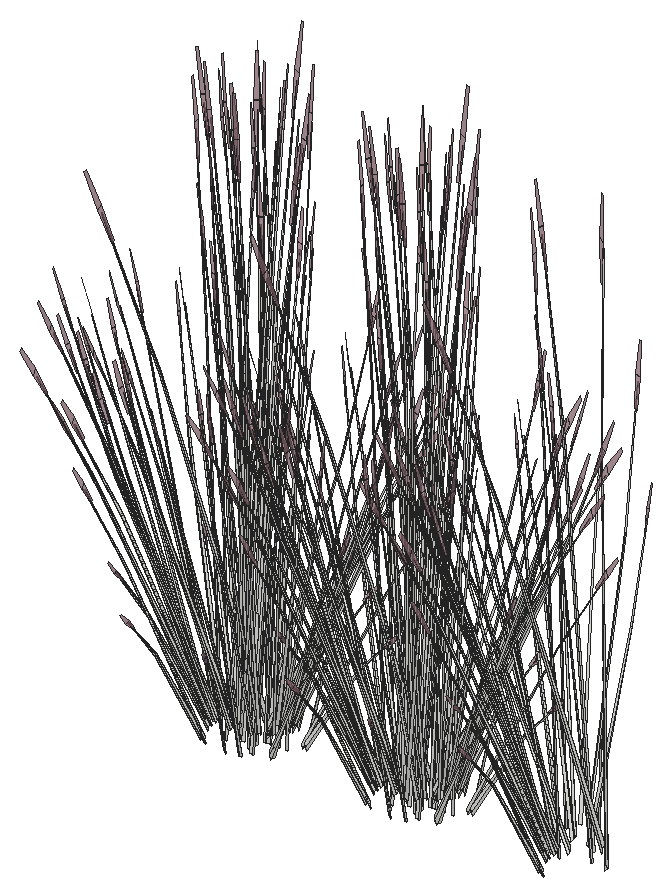
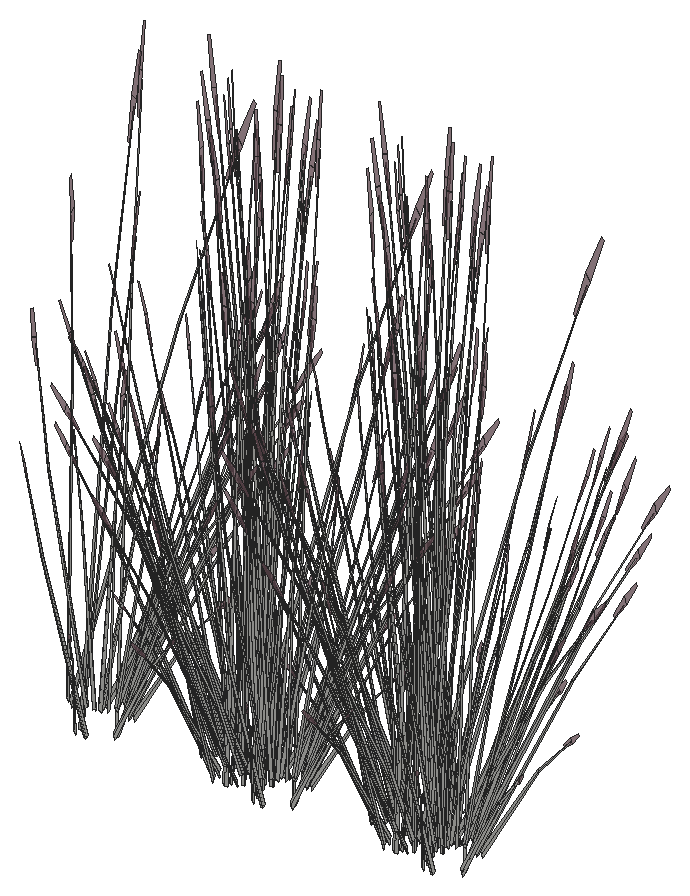
# SketchUp Ruby script. Lengths in inches.
U = 1.inch
M = Sketchup.active_model
def pt(a) = Geom::Point3d.new(a.map { |v| v * U })
def face(e, loops, mat)
  f = e.add_face(loops[0].map { |a| pt(a) })
  loops[1..].each { |l| e.add_face(l.map { |a| pt(a) }).erase! }
  f.material = f.back_material = mat if mat
  f
end
# faces: each face lists its corners as indices into pts; further lists are holes
def faces(e, pts, list, mat = nil) = list.each { |f| face(e, (f[0].is_a?(Array) ? f : [f]).map { |l| l.map { |i| pts[i] } }, mat) }
# xy, xz, yz: faces in a plane at the given z, y or x. An outline is a flat list of corners, or four numbers for a rectangle; further outlines are holes
def ring(l) = l.size == 4 ? [[l[0], l[1]], [l[2], l[1]], [l[2], l[3]], [l[0], l[3]]] : l.each_slice(2).to_a
def flat(e, list, mat, &to3) = list.each { |f| face(e, (f[0].is_a?(Array) ? f : [f]).map { |l| ring(l).map { |u, v| to3.(u, v) } }, mat) }
def xy(e, z, list, mat = nil) = flat(e, list, mat) { |x, y| [x, y, z] }
def xz(e, y, list, mat = nil) = flat(e, list, mat) { |x, z| [x, y, z] }
def yz(e, x, list, mat = nil) = flat(e, list, mat) { |y, z| [x, y, z] }
def lines(e, pts, list) = list.each { |a, b| e.add_line(pt(pts[a]), pt(pts[b])) }
# prism: a flat outline (further loops are holes) pulled along v
def prism(e, loops, v, mat = nil)
  f = face(e, loops, mat); d = Geom::Vector3d.new(v.map { |x| x * U })
  f.pushpull(f.normal.samedirection?(d) ? d.length : -d.length)
end
def box(e, o, s, mat = nil) = prism(e, [[o, [o[0] + s[0], o[1], o[2]], [o[0] + s[0], o[1] + s[1], o[2]], [o[0], o[1] + s[1], o[2]]]], [0, 0, s[2]], mat)
def at(x, y, z, deg = 0) = Geom::Transformation.translation(pt([x, y, z])) * Geom::Transformation.rotation(ORIGIN, Z_AXIS, deg.degrees)
def axes(o, x, y, z) = Geom::Transformation.new([*x, 0, *y, 0, *z, 0, *pt(o).to_a, 1])
def part(name) = M.definitions.add(name)
# library, detail: a bought-in or finely detailed component or shape, given as its bounding box
def library(name, o, s) = part(name).tap { |d| box(d.entities, o, s) }
def detail(e, o, s) = box(e.add_group.entities, o, s)
def put(e, d, t, mat = nil) = e.add_instance(d, t).tap { |i| i.material = mat if mat }
def group(e, t, mat = nil) = e.add_group.tap { |g| g.transformation = t; g.material = mat if mat }.entities
root = M.entities
M.materials.add("LightPink_Translucent").color = [144, 107, 117]
M.materials["LightPink_Translucent"].alpha = 0.75
c1 = part("blade")
p = [[2.15,0.21,22],[0,0.17,0],[0.09,0.45,0],[2.18,0.31,22],[2.29,0.31,22],[0.38,0.45,0],
  [2.48,0.24,33],[2.49,0.24,33],[2.48,0.22,33]]
faces(c1.entities,p,[[0,1,2,3],[4,5,2,3],[6,3,4,7],[8,0,3,6]])
c2 = part("seeds")
p = [[0.3,-0.1,1.38],[-0.01,-0.03,1.59],[-0.01,-0.03,0.03],[0.14,-0.07,-0.07],[0.29,-0.03,3],[0.15,0.01,3.11]]
faces(c2.entities,p,[[0,1,2,3],[1,0,4,5]],"LightPink_Translucent")
c3 = part("blade with seeds")
put(c3.entities,c1,at(0,0,0))
put(c3.entities,c2,axes([2.4,0.25,30.99],[1.5799,-0.05474,1.17369],[-0.12525,1.92788,0.29478],[-0.07173,-0.02425,1.56792]))
put(root,c3,axes([242.36,52.72,258.875],[0.31515,-0.01384,1.71376],[-0.20907,0.5998,0.13857],[-0.44912,-0.0371,0.73262]))
put(root,c3,axes([242.49,53.77,258.875],[0.26363,-0.12925,1.71376],[0.22195,0.59723,0.13857],[-0.41388,0.13498,0.73262]))
put(root,c3,axes([241.67,54.79,257.59],[0.26405,0.05016,1.43002],[0.17019,0.51235,-0.30754],[-0.35868,0.0959,0.61141]))
put(root,c3,axes([244,53.15,258.34],[0.21597,-0.08839,1.77064],[0.07448,0.61717,0.13857],[-0.4678,0.08189,0.63284]))
put(root,c3,axes([243.3,52.16,259.98],[-0.75952,-0.01471,-0.71045],[0.05101,-0.61953,0.08574],[-0.32177,-0.06538,1.00501]))
put(root,c3,axes([242.6875,52.31,257.59],[0.14835,0.17012,1.43002],[-0.34183,0.46242,-0.30754],[-0.351,-0.11053,0.61141]))
put(root,c3,axes([242.08,53.23,259.53],[-0.63144,-0.17046,-0.35414],[0.18417,-0.49731,0.4572],[-0.25423,0.0456,0.87481]))
put(root,c3,axes([242.95,51.75,258.875],[0.28223,0.10528,1.71376],[-0.58406,0.44165,0.13857],[-0.36402,-0.19924,0.73262]))
put(root,c3,axes([242.51,53.49,259.68],[-0.20584,0.55581,-0.51099],[-0.70573,-0.19051,-0.3958],[-0.28414,0.05097,0.97773]))
put(root,c3,axes([243.05,52.28,259.68],[-0.55171,0.40476,-0.51099],[-0.48318,-0.42758,-0.3958],[-0.28031,-0.06159,0.97773]))
put(root,c3,axes([241.12,55.86,257.77],[0.31665,-0.27694,1.1486],[0.12495,0.43841,0.84392],[-0.22883,0.0785,0.25299]))
put(root,c3,axes([242.84,51.9,259.53],[-0.43232,-0.38257,-0.35414],[0.49364,-0.36215,0.4572],[-0.25081,-0.0551,0.87481]))
put(root,c3,axes([243.45,54.17,258.875],[0.18977,-0.18775,1.71376],[0.47917,0.50677,0.13857],[-0.32866,0.23079,0.73262]))
put(root,c3,axes([242.3125,54.67,259.53],[-0.66138,0.08733,-0.35414],[-0.17464,-0.49921,0.4572],[-0.18953,0.13408,0.87481]))
put(root,c3,axes([241.81,52.82,257.77],[0.48508,-0.04372,1.1486],[-0.3077,0.38525,0.84392],[-0.23971,-0.05779,0.25299]))
put(root,c3,axes([243.3125,54.64,258.875],[0.14147,-0.21002,1.71376],[0.59349,0.43464,0.13857],[-0.26773,0.27089,0.73262]))
put(root,c3,axes([242.86,54.72,259.68],[0.19519,0.55794,-0.51099],[-0.73919,0.0976,-0.3958],[-0.21183,0.14986,0.97773]))
put(root,c3,axes([244.62,51.43,259.98],[-0.64788,-0.29534,-0.71045],[0.46044,-0.51755,0.08574],[-0.23473,-0.17635,1.00501]))
put(root,c3,axes([244.32,51.44,259.68],[-0.74975,0.14525,-0.51099],[-0.13115,-0.55007,-0.3958],[-0.20138,-0.15763,0.97773]))
put(root,c3,axes([243.9,50.625,257.59],[-0.04601,0.19989,1.43002],[-0.67263,0.16733,-0.30754],[-0.15723,-0.25836,0.61141]))
put(root,c3,axes([244.12,51.14,258.875],[0.17368,0.19618,1.71376],[-0.80256,0.16516,0.13857],[-0.18139,-0.30799,0.73262]))
put(root,c3,axes([244.4,51.04,259.53],[-0.11735,-0.49217,-0.35414],[0.67083,-0.12996,0.4572],[-0.18018,-0.14104,0.87481]))
put(root,c3,axes([243.48,55.82,259.53],[-0.5141,0.32171,-0.35414],[-0.48666,-0.36734,0.4572],[-0.07405,0.18664,0.87481]))
put(root,c3,axes([246.17,54.77,258.33],[0.65659,0.2464,1.51261],[-0.64324,0.53082,0.59816],[-0.28812,-0.31461,1.26806]))
put(root,c3,axes([243.67,50.3,257.77],[0.39634,0.21267,1.1486],[-0.57721,0.12784,0.84392],[-0.1235,-0.16344,0.25299]))
put(root,c3,axes([243.8,57.07,257.77],[-0.01966,-0.36332,1.1486],[0.49135,0.25914,0.84392],[-0.09663,0.17317,0.25299]))
put(root,c3,axes([244.51,55.54,257.48],[0.7111,0.30552,0.49651],[-0.42504,0.54784,0],[-0.16196,-0.06958,1.57504]))
put(root,c3,axes([245.52,54.59,257.62],[-0.14658,0.54532,0.1448],[-0.71613,-0.09466,-0.41347],[-0.13033,-0.05599,1.26744]))
put(root,c3,axes([243.1,53.63,257.48],[0,0.61104,0.49651],[-0.85008,0,0],[0,-0.13917,1.57504]))
put(root,c3,axes([243.99,55.67,260],[0.54391,0.41056,-0.5672],[-0.57458,0.35956,-0.43934],[-0.08276,0.2086,1.08528]))
put(root,c3,axes([247.19,53.59,257.84],[-0.02076,-0.57531,1.41272],[0.93937,0.14913,0.59816],[-0.22217,0.31481,1.3335]))
put(root,c3,axes([243.4,56.29,257.82],[0.69024,-0.1082,0.06507],[0.15868,0.43593,-0.86304],[-0.04376,0.22067,0.7736]))
put(root,c3,axes([245.98,51.1875,259.68],[-0.7469,-0.15318,-0.51099],[0.25601,-0.52518,-0.3958],[-0.06849,-0.21144,0.97773]))
put(root,c3,axes([245.29,54.07,257.36],[0.96033,0.12874,0.45755],[-0.19544,0.7271,0.17955],[-0.14034,-0.07021,1.58856]))
put(root,c3,axes([245.04,53.94,257.72],[-0.36864,0.55059,0.44739],[-0.76598,-0.26498,-0.21531],[0,-0.12692,1.43643]))
put(root,c3,axes([246.26,51.29,259.98],[-0.36264,-0.49684,-0.71045],[0.74649,-0.27689,0.08574],[-0.0848,-0.24006,1.00501]))
put(root,c3,axes([244.77,55.23,257.47],[0.81646,-0.16218,0.17642],[0.20161,0.60355,0.35086],[-0.07282,-0.08794,1.60407]))
put(root,c3,axes([247.2,55.27,257.47],[0.21949,-0.60727,0.17642],[0.8032,0.17185,0.35086],[-0.13875,0.00296,1.60407]))
put(root,c3,axes([246.83,54.46,257.62],[0.56134,0.36712,0.1448],[-0.46823,0.41419,-0.41347],[-0.13033,0.05599,1.26744]))
put(root,c3,axes([246.82,54.19,257.72],[0.82508,-0.03772,0.44739],[0.07462,0.62614,-0.21531],[-0.14771,0.06346,1.43643]))
put(root,c3,axes([247.43,55.59,257.48],[0.7111,-0.30552,0.49651],[0.42504,0.54784,0],[-0.16196,0.06958,1.57504]))
put(root,c3,axes([246.32,50.87,259.53],[0.22906,-0.4699,-0.35414],[0.66828,0.13705,0.4572],[-0.06128,-0.18919,0.87481]))
put(root,c3,axes([245.21,53.4,257.36],[0.33034,0.68327,0.45755],[-0.94388,0.2376,0.17955],[0.01154,-0.12555,1.58856]))
put(root,c3,axes([248.46,53.72,257.47],[-0.59697,-0.44509,0.17642],[0.60159,-0.4317,0.35086],[-0.06593,0.0909,1.60407]))
put(root,c3,axes([245.51,53.59,257.43],[0.8561,0.29616,0.24065],[-0.41201,0.61537,0.50002],[0,-0.14185,1.60543]))
put(root,c3,axes([245.23,53.18,257.72],[-0.82508,0.03772,0.44739],[-0.07462,-0.62614,-0.21531],[0.14771,-0.06346,1.43643]))
put(root,c3,axes([244.85,52.1,257.47],[-0.21949,0.60727,0.17642],[-0.8032,-0.17185,0.35086],[0.13875,-0.00296,1.60407]))
put(root,c3,axes([247.28,52.14,257.47],[-0.81646,0.16218,0.17642],[-0.20161,-0.60355,0.35086],[0.07282,0.08794,1.60407]))
put(root,c3,axes([246.45,49.875,257.77],[0.09747,0.35631,1.1486],[-0.54071,-0.19735,0.84392],[0.05818,-0.18244,0.25299]))
put(root,c3,axes([245.94,53.02,257.36],[-0.62999,0.55453,0.45755],[-0.74845,-0.4895,0.17955],[0.15188,-0.05534,1.58856]))
put(root,c3,axes([247.01,53.43,257.72],[0.36864,-0.55059,0.44739],[0.76598,0.26498,-0.21531],[0,0.12692,1.43643]))
put(root,c3,axes([245.6,56.07,259.68],[0.7469,0.15318,-0.51099],[-0.25601,0.52518,-0.3958],[0.06849,0.21144,0.97773]))
put(root,c3,axes([246.76,53.3,257.38],[-0.96033,-0.12874,0.49198],[0.19544,-0.7271,0.19306],[0.14034,0.07021,1.70813]))
put(root,c3,axes([246.22,52.92,257.72],[-0.45644,-0.51287,0.44739],[0.69137,-0.36116,-0.21531],[0.14771,0.06346,1.43643]))
put(root,c3,axes([247.33,53.55,257.62],[0.70791,-0.1782,0.1448],[0.24791,0.50885,-0.41347],[0,0.11199,1.26744]))
put(root,c3,axes([247.6,51.59,259.68],[-0.54391,-0.41056,-0.51099],[0.57458,-0.35956,-0.3958],[0.08276,-0.2086,0.97773]))
put(root,c3,axes([247.24,50.86,257.59],[-0.21597,0.12368,1.43002],[-0.64681,-0.21647,-0.30754],[0.1199,-0.26922,0.61141]))
put(root,c3,axes([248.95,53.74,257.48],[0,-0.61104,0.49651],[0.85008,0,0],[0,0.13917,1.57504]))
put(root,c3,axes([246.53,52.78,257.62],[0.14658,-0.54532,0.1448],[0.71613,0.09466,-0.41347],[0.13033,0.05599,1.26744]))
put(root,c3,axes([247.55,51.83,257.48],[-0.7111,-0.30552,0.49651],[0.42504,-0.54784,0],[0.16196,0.06958,1.57504]))
put(root,c3,axes([247.77,51.77,259.98],[0.01977,-0.56521,-0.71045],[0.83252,0.03796,0.08574],[0.08786,-0.23945,1.00501]))
put(root,c3,axes([248.11,51.43,259.53],[0.5141,-0.32171,-0.35414],[0.48666,0.36734,0.4572],[0.07405,-0.18664,0.87481]))
put(root,c3,axes([248.23,55.57,257.77],[-0.4278,-0.1757,1.1486],[0.5524,-0.17852,0.84392],[0.14899,0.15122,0.25299]))
put(root,c3,axes([246.71,55.38,257.59],[0.01341,-0.20255,1.43002],[0.64074,-0.22625,-0.30754],[0.1978,0.24243,0.61141]))
put(root,c3,axes([258.42,52.72,258.875],[0.31515,-0.01384,1.71376],[-0.20907,0.5998,0.13857],[-0.44912,-0.0371,0.73262]))
put(root,c3,axes([248.3,56.37,257.67],[-0.48723,-0.01916,1.0506],[0.32177,-0.40701,0.58006],[0.19248,0.1446,0.8241]))
put(root,c3,axes([246.83,51.49,258.875],[-0.14147,0.21002,1.71376],[-0.59349,-0.43464,0.13857],[0.26773,-0.27089,0.73262]))
put(root,c3,axes([258.56,53.77,258.875],[0.26363,-0.12925,1.71376],[0.22195,0.59723,0.13857],[-0.41388,0.13498,0.73262]))
put(root,c3,axes([257.73,54.79,257.59],[0.26405,0.05016,1.43002],[0.17019,0.51235,-0.30754],[-0.35868,0.0959,0.61141]))
put(root,c3,axes([260.07,53.15,258.34],[0.21597,-0.08839,1.77064],[0.07448,0.61717,0.13857],[-0.4678,0.08189,0.63284]))
put(root,c3,axes([247.27,55.8125,259.68],[0.74975,-0.14525,-0.51099],[0.13115,0.55007,-0.3958],[0.20138,0.15763,0.97773]))
put(root,c3,axes([248.73,52.53,259.68],[-0.19519,-0.55794,-0.51099],[0.73919,-0.0976,-0.3958],[0.21183,-0.14986,0.97773]))
put(root,c3,axes([259.37,52.16,259.98],[-0.75952,-0.01471,-0.71045],[0.05101,-0.61953,0.08574],[-0.32177,-0.06538,1.00501]))
put(root,c3,axes([258.75,52.31,257.59],[0.14835,0.17012,1.43002],[-0.34183,0.46242,-0.30754],[-0.351,-0.11053,0.61141]))
put(root,c3,axes([250.03,55.41,258.93],[-0.14542,-0.51365,-0.03492],[0.68734,-0.11809,-0.15832],[0.14353,0.03256,0.52218]))
put(root,c3,axes([258.15,53.23,259.53],[-0.63144,-0.17046,-0.35414],[0.18417,-0.49731,0.4572],[-0.25423,0.0456,0.87481]))
put(root,c3,axes([259.02,51.75,258.875],[0.28223,0.10528,1.71376],[-0.58406,0.44165,0.13857],[-0.36402,-0.19924,0.73262]))
put(root,c3,axes([258.58,53.49,259.68],[-0.20584,0.55581,-0.51099],[-0.70573,-0.19051,-0.3958],[-0.28414,0.05097,0.97773]))
put(root,c3,axes([249.63,51.42,257.77],[-0.25308,0.31105,1.1486],[-0.21753,-0.4179,0.84392],[0.20902,-0.10472,0.25299]))
put(root,c3,axes([259.11,52.28,259.68],[-0.55171,0.40476,-0.51099],[-0.48318,-0.42758,-0.3958],[-0.28031,-0.06159,0.97773]))
put(root,c3,axes([247.1875,54.37,258.875],[-0.28223,-0.10528,1.71376],[0.58406,-0.44165,0.13857],[0.36402,0.19924,0.73262]))
put(root,c3,axes([257.18,55.86,257.77],[0.31665,-0.27694,1.1486],[0.12495,0.43841,0.84392],[-0.22883,0.0785,0.25299]))
put(root,c3,axes([249.27,52.59,259.53],[0.66138,-0.08733,-0.35414],[0.17464,0.49921,0.4572],[0.18953,-0.13408,0.87481]))
put(root,c3,axes([248.75,52.76,259.98],[0.39688,-0.48213,-0.71045],[0.69548,0.34264,0.08574],[0.23697,-0.17468,1.00501]))
put(root,c3,axes([248.74,55.35,259.53],[0.43232,0.38257,-0.35414],[-0.49364,0.36215,0.4572],[0.25081,0.0551,0.87481]))
put(root,c3,axes([258.91,51.9,259.53],[-0.43232,-0.38257,-0.35414],[0.49364,-0.36215,0.4572],[-0.25081,-0.0551,0.87481]))
put(root,c3,axes([259.52,54.17,258.875],[0.18977,-0.18775,1.71376],[0.47917,0.50677,0.13857],[-0.32866,0.23079,0.73262]))
put(root,c3,axes([258.38,54.67,259.53],[-0.66138,0.08733,-0.35414],[-0.17464,-0.49921,0.4572],[-0.18953,0.13408,0.87481]))
put(root,c3,axes([257.87,52.82,257.77],[0.48508,-0.04372,1.1486],[-0.3077,0.38525,0.84392],[-0.23971,-0.05779,0.25299]))
put(root,c3,axes([249.07,53.77,259.68],[0.20584,-0.55581,-0.51099],[0.70573,0.19051,-0.3958],[0.28414,-0.05097,0.97773]))
put(root,c3,axes([250.84,54.125,257.77],[-0.46945,0.10088,1.1486],[0.22097,-0.4169,0.84392],[0.24904,0.02853,0.25299]))
put(root,c3,axes([259.38,54.64,258.875],[0.14147,-0.21002,1.71376],[0.59349,0.43464,0.13857],[-0.26773,0.27089,0.73262]))
put(root,c3,axes([249.32,52.3125,257.59],[-0.27143,-0.0181,1.43002],[-0.27808,-0.48551,-0.30754],[0.33346,-0.13735,0.61141]))
put(root,c3,axes([249.5,54.02,259.53],[0.63144,0.17046,-0.35414],[-0.18417,0.49731,0.4572],[0.25423,-0.0456,0.87481]))
put(root,c3,axes([248.28,55.1,259.98],[0.75952,0.01471,-0.71045],[-0.05101,0.61953,0.08574],[0.32177,0.06538,1.00501]))
put(root,c3,axes([258.92,54.72,259.68],[0.19519,0.55794,-0.51099],[-0.73919,0.0976,-0.3958],[-0.21183,0.14986,0.97773]))
put(root,c3,axes([247.78,53.41,258.875],[-0.31515,0.01384,1.71376],[0.20907,-0.5998,0.13857],[0.44912,0.0371,0.73262]))
put(root,c3,axes([260.6875,51.43,259.98],[-0.64788,-0.29534,-0.71045],[0.46044,-0.51755,0.08574],[-0.23473,-0.17635,1.00501]))
put(root,c3,axes([260.38,51.44,259.68],[-0.74975,0.14525,-0.51099],[-0.13115,-0.55007,-0.3958],[-0.20138,-0.15763,0.97773]))
put(root,c3,axes([248.9375,53.97,259.98],[0.66765,-0.26986,-0.71045],[0.37208,0.55551,0.08574],[0.32259,-0.0631,1.00501]))
put(root,c3,axes([249.96,54.79,257.59],[-0.18299,-0.15028,1.43002],[0.23809,-0.49714,-0.30754],[0.37023,0.06735,0.61141]))
put(root,c3,axes([259.96,50.625,257.59],[-0.04601,0.19989,1.43002],[-0.67263,0.16733,-0.30754],[-0.15723,-0.25836,0.61141]))
put(root,c3,axes([260.18,51.14,258.875],[0.17368,0.19618,1.71376],[-0.80256,0.16516,0.13857],[-0.18139,-0.30799,0.73262]))
put(root,c3,axes([260.46,51.04,259.53],[-0.11735,-0.49217,-0.35414],[0.67083,-0.12996,0.4572],[-0.18018,-0.14104,0.87481]))
put(root,c3,axes([259.54,55.82,259.53],[-0.5141,0.32171,-0.35414],[-0.48666,-0.36734,0.4572],[-0.07405,0.18664,0.87481]))
put(root,c3,axes([262.24,54.77,258.33],[0.65659,0.2464,1.51261],[-0.64324,0.53082,0.59816],[-0.28812,-0.31461,1.26806]))
put(root,c3,axes([259.73,50.3,257.77],[0.39634,0.21267,1.1486],[-0.57721,0.12784,0.84392],[-0.1235,-0.16344,0.25299]))
put(root,c3,axes([259.87,57.07,257.77],[-0.01966,-0.36332,1.1486],[0.49135,0.25914,0.84392],[-0.09663,0.17317,0.25299]))
put(root,c3,axes([260.57,55.54,257.48],[0.7111,0.30552,0.49651],[-0.42504,0.54784,0],[-0.16196,-0.06958,1.57504]))
put(root,c3,axes([261.59,54.59,257.62],[-0.14658,0.54532,0.1448],[-0.71613,-0.09466,-0.41347],[-0.13033,-0.05599,1.26744]))
put(root,c3,axes([259.17,53.63,257.48],[0,0.61104,0.49651],[-0.85008,0,0],[0,-0.13917,1.57504]))
put(root,c3,axes([260.05,55.67,260],[0.54391,0.41056,-0.5672],[-0.57458,0.35956,-0.43934],[-0.08276,0.2086,1.08528]))
put(root,c3,axes([263.26,53.59,257.84],[-0.02076,-0.57531,1.41272],[0.93937,0.14913,0.59816],[-0.22217,0.31481,1.3335]))
put(root,c3,axes([259.46,56.29,257.82],[0.69024,-0.1082,0.06507],[0.15868,0.43593,-0.86304],[-0.04376,0.22067,0.7736]))
put(root,c3,axes([262.05,51.1875,259.68],[-0.7469,-0.15318,-0.51099],[0.25601,-0.52518,-0.3958],[-0.06849,-0.21144,0.97773]))
put(root,c3,axes([261.35,54.07,257.36],[0.96033,0.12874,0.45755],[-0.19544,0.7271,0.17955],[-0.14034,-0.07021,1.58856]))
put(root,c3,axes([261.1,53.94,257.72],[-0.36864,0.55059,0.44739],[-0.76598,-0.26498,-0.21531],[0,-0.12692,1.43643]))
put(root,c3,axes([262.32,51.29,259.98],[-0.36264,-0.49684,-0.71045],[0.74649,-0.27689,0.08574],[-0.0848,-0.24006,1.00501]))
put(root,c3,axes([260.84,55.23,257.47],[0.81646,-0.16218,0.17642],[0.20161,0.60355,0.35086],[-0.07282,-0.08794,1.60407]))
put(root,c3,axes([263.27,55.27,257.47],[0.21949,-0.60727,0.17642],[0.8032,0.17185,0.35086],[-0.13875,0.00296,1.60407]))
put(root,c3,axes([262.9,54.46,257.62],[0.56134,0.36712,0.1448],[-0.46823,0.41419,-0.41347],[-0.13033,0.05599,1.26744]))
put(root,c3,axes([262.88,54.19,257.72],[0.82508,-0.03772,0.44739],[0.07462,0.62614,-0.21531],[-0.14771,0.06346,1.43643]))
put(root,c3,axes([263.49,55.59,257.48],[0.7111,-0.30552,0.49651],[0.42504,0.54784,0],[-0.16196,0.06958,1.57504]))
put(root,c3,axes([262.39,50.87,259.53],[0.22906,-0.4699,-0.35414],[0.66828,0.13705,0.4572],[-0.06128,-0.18919,0.87481]))
put(root,c3,axes([261.27,53.4,257.36],[0.33034,0.68327,0.45755],[-0.94388,0.2376,0.17955],[0.01154,-0.12555,1.58856]))
put(root,c3,axes([264.52,53.72,257.47],[-0.59697,-0.44509,0.17642],[0.60159,-0.4317,0.35086],[-0.06593,0.0909,1.60407]))
put(root,c3,axes([261.58,53.59,257.43],[0.8561,0.29616,0.24065],[-0.41201,0.61537,0.50002],[0,-0.14185,1.60543]))
put(root,c3,axes([261.3,53.18,257.72],[-0.82508,0.03772,0.44739],[-0.07462,-0.62614,-0.21531],[0.14771,-0.06346,1.43643]))
put(root,c3,axes([260.91,52.1,257.47],[-0.21949,0.60727,0.17642],[-0.8032,-0.17185,0.35086],[0.13875,-0.00296,1.60407]))
put(root,c3,axes([263.34,52.14,257.47],[-0.81646,0.16218,0.17642],[-0.20161,-0.60355,0.35086],[0.07282,0.08794,1.60407]))
put(root,c3,axes([262.51,49.875,257.77],[0.09747,0.35631,1.1486],[-0.54071,-0.19735,0.84392],[0.05818,-0.18244,0.25299]))
put(root,c3,axes([262.01,53.02,257.36],[-0.62999,0.55453,0.45755],[-0.74845,-0.4895,0.17955],[0.15188,-0.05534,1.58856]))
put(root,c3,axes([263.08,53.43,257.72],[0.36864,-0.55059,0.44739],[0.76598,0.26498,-0.21531],[0,0.12692,1.43643]))
put(root,c3,axes([261.67,56.07,259.68],[0.7469,0.15318,-0.51099],[-0.25601,0.52518,-0.3958],[0.06849,0.21144,0.97773]))
put(root,c3,axes([262.83,53.3,257.38],[-0.96033,-0.12874,0.49198],[0.19544,-0.7271,0.19306],[0.14034,0.07021,1.70813]))
put(root,c3,axes([262.29,52.92,257.72],[-0.45644,-0.51287,0.44739],[0.69137,-0.36116,-0.21531],[0.14771,0.06346,1.43643]))
put(root,c3,axes([263.4,53.55,257.62],[0.70791,-0.1782,0.1448],[0.24791,0.50885,-0.41347],[0,0.11199,1.26744]))
put(root,c3,axes([263.66,51.59,259.68],[-0.54391,-0.41056,-0.51099],[0.57458,-0.35956,-0.3958],[0.08276,-0.2086,0.97773]))
put(root,c3,axes([263.31,50.86,257.59],[-0.21597,0.12368,1.43002],[-0.64681,-0.21647,-0.30754],[0.1199,-0.26922,0.61141]))
put(root,c3,axes([265.01,53.74,257.48],[0,-0.61104,0.49651],[0.85008,0,0],[0,0.13917,1.57504]))
put(root,c3,axes([262.09,54.98,258.875],[-0.17368,-0.19618,1.71376],[0.80256,-0.16516,0.13857],[0.18139,0.30799,0.73262]))
put(root,c3,axes([262.59,52.78,257.62],[0.14658,-0.54532,0.1448],[0.71613,0.09466,-0.41347],[0.13033,0.05599,1.26744]))
put(root,c3,axes([263.61,51.83,257.48],[-0.7111,-0.30552,0.49651],[0.42504,-0.54784,0],[0.16196,0.06958,1.57504]))
put(root,c3,axes([263.83,51.77,259.98],[0.01977,-0.56521,-0.71045],[0.83252,0.03796,0.08574],[0.08786,-0.23945,1.00501]))
put(root,c3,axes([264.17,51.43,259.53],[0.5141,-0.32171,-0.35414],[0.48666,0.36734,0.4572],[0.07405,-0.18664,0.87481]))
put(root,c3,axes([264.3,55.57,257.77],[-0.4278,-0.1757,1.1486],[0.5524,-0.17852,0.84392],[0.14899,0.15122,0.25299]))
put(root,c3,axes([262.77,55.38,257.59],[0.01341,-0.20255,1.43002],[0.64074,-0.22625,-0.30754],[0.1978,0.24243,0.61141]))
put(root,c3,axes([264.37,56.37,257.67],[-0.48723,-0.01916,1.0506],[0.32177,-0.40701,0.58006],[0.19248,0.1446,0.8241]))
put(root,c3,axes([262.89,51.49,258.875],[-0.14147,0.21002,1.71376],[-0.59349,-0.43464,0.13857],[0.26773,-0.27089,0.73262]))
put(root,c3,axes([275.15,52.72,258.875],[0.31515,-0.01384,1.71376],[-0.20907,0.5998,0.13857],[-0.44912,-0.0371,0.73262]))
put(root,c3,axes([263.33,55.8125,259.68],[0.74975,-0.14525,-0.51099],[0.13115,0.55007,-0.3958],[0.20138,0.15763,0.97773]))
put(root,c3,axes([275.28,53.77,258.875],[0.26363,-0.12925,1.71376],[0.22195,0.59723,0.13857],[-0.41388,0.13498,0.73262]))
put(root,c3,axes([274.46,54.79,257.59],[0.26405,0.05016,1.43002],[0.17019,0.51235,-0.30754],[-0.35868,0.0959,0.61141]))
put(root,c3,axes([264.79,52.53,259.68],[-0.19519,-0.55794,-0.51099],[0.73919,-0.0976,-0.3958],[0.21183,-0.14986,0.97773]))
put(root,c3,axes([266.09,55.41,258.93],[-0.14542,-0.51365,-0.03492],[0.68734,-0.11809,-0.15832],[0.14353,0.03256,0.52218]))
put(root,c3,axes([276.8,53.15,258.34],[0.21597,-0.08839,1.77064],[0.07448,0.61717,0.13857],[-0.4678,0.08189,0.63284]))
put(root,c3,axes([265.7,51.42,257.77],[-0.25308,0.31105,1.1486],[-0.21753,-0.4179,0.84392],[0.20902,-0.10472,0.25299]))
put(root,c3,axes([276.1,52.16,259.98],[-0.75952,-0.01471,-0.71045],[0.05101,-0.61953,0.08574],[-0.32177,-0.06538,1.00501]))
put(root,c3,axes([275.48,52.31,257.59],[0.14835,0.17012,1.43002],[-0.34183,0.46242,-0.30754],[-0.351,-0.11053,0.61141]))
put(root,c3,axes([274.875,53.23,259.53],[-0.63144,-0.17046,-0.35414],[0.18417,-0.49731,0.4572],[-0.25423,0.0456,0.87481]))
put(root,c3,axes([275.75,51.75,258.875],[0.28223,0.10528,1.71376],[-0.58406,0.44165,0.13857],[-0.36402,-0.19924,0.73262]))
put(root,c3,axes([263.25,54.37,258.875],[-0.28223,-0.10528,1.71376],[0.58406,-0.44165,0.13857],[0.36402,0.19924,0.73262]))
put(root,c3,axes([275.31,53.49,259.68],[-0.20584,0.55581,-0.51099],[-0.70573,-0.19051,-0.3958],[-0.28414,0.05097,0.97773]))
put(root,c3,axes([265.34,52.59,259.53],[0.66138,-0.08733,-0.35414],[0.17464,0.49921,0.4572],[0.18953,-0.13408,0.87481]))
put(root,c3,axes([264.8125,52.76,259.98],[0.39688,-0.48213,-0.71045],[0.69548,0.34264,0.08574],[0.23697,-0.17468,1.00501]))
put(root,c3,axes([264.81,55.35,259.53],[0.43232,0.38257,-0.35414],[-0.49364,0.36215,0.4572],[0.25081,0.0551,0.87481]))
put(root,c3,axes([275.84,52.28,259.68],[-0.55171,0.40476,-0.51099],[-0.48318,-0.42758,-0.3958],[-0.28031,-0.06159,0.97773]))
put(root,c3,axes([273.91,55.86,257.77],[0.31665,-0.27694,1.1486],[0.12495,0.43841,0.84392],[-0.22883,0.0785,0.25299]))
put(root,c3,axes([275.64,51.9,259.53],[-0.43232,-0.38257,-0.35414],[0.49364,-0.36215,0.4572],[-0.25081,-0.0551,0.87481]))
put(root,c3,axes([276.25,54.17,258.875],[0.18977,-0.18775,1.71376],[0.47917,0.50677,0.13857],[-0.32866,0.23079,0.73262]))
put(root,c3,axes([275.11,54.67,259.53],[-0.66138,0.08733,-0.35414],[-0.17464,-0.49921,0.4572],[-0.18953,0.13408,0.87481]))
put(root,c3,axes([265.14,53.77,259.68],[0.20584,-0.55581,-0.51099],[0.70573,0.19051,-0.3958],[0.28414,-0.05097,0.97773]))
put(root,c3,axes([266.91,54.125,257.77],[-0.46945,0.10088,1.1486],[0.22097,-0.4169,0.84392],[0.24904,0.02853,0.25299]))
put(root,c3,axes([274.6,52.82,257.77],[0.48508,-0.04372,1.1486],[-0.3077,0.38525,0.84392],[-0.23971,-0.05779,0.25299]))
put(root,c3,axes([265.39,52.3125,257.59],[-0.27143,-0.0181,1.43002],[-0.27808,-0.48551,-0.30754],[0.33346,-0.13735,0.61141]))
put(root,c3,axes([265.57,54.02,259.53],[0.63144,0.17046,-0.35414],[-0.18417,0.49731,0.4572],[0.25423,-0.0456,0.87481]))
put(root,c3,axes([264.35,55.1,259.98],[0.75952,0.01471,-0.71045],[-0.05101,0.61953,0.08574],[0.32177,0.06538,1.00501]))
put(root,c3,axes([263.85,53.41,258.875],[-0.31515,0.01384,1.71376],[0.20907,-0.5998,0.13857],[0.44912,0.0371,0.73262]))
put(root,c3,axes([276.11,54.64,258.875],[0.14147,-0.21002,1.71376],[0.59349,0.43464,0.13857],[-0.26773,0.27089,0.73262]))
put(root,c3,axes([265,53.97,259.98],[0.66765,-0.26986,-0.71045],[0.37208,0.55551,0.08574],[0.32259,-0.0631,1.00501]))
put(root,c3,axes([275.65,54.72,259.68],[0.19519,0.55794,-0.51099],[-0.73919,0.0976,-0.3958],[-0.21183,0.14986,0.97773]))
put(root,c3,axes([277.42,51.43,259.98],[-0.64788,-0.29534,-0.71045],[0.46044,-0.51755,0.08574],[-0.23473,-0.17635,1.00501]))
put(root,c3,axes([277.11,51.44,259.68],[-0.74975,0.14525,-0.51099],[-0.13115,-0.55007,-0.3958],[-0.20138,-0.15763,0.97773]))
put(root,c3,axes([266.03,54.79,257.59],[-0.18299,-0.15028,1.43002],[0.23809,-0.49714,-0.30754],[0.37023,0.06735,0.61141]))
put(root,c3,axes([276.69,50.625,257.59],[-0.04601,0.19989,1.43002],[-0.67263,0.16733,-0.30754],[-0.15723,-0.25836,0.61141]))
put(root,c3,axes([276.91,51.14,258.875],[0.17368,0.19618,1.71376],[-0.80256,0.16516,0.13857],[-0.18139,-0.30799,0.73262]))
put(root,c3,axes([277.19,51.04,259.53],[-0.11735,-0.49217,-0.35414],[0.67083,-0.12996,0.4572],[-0.18018,-0.14104,0.87481]))
put(root,c3,axes([276.27,55.82,259.53],[-0.5141,0.32171,-0.35414],[-0.48666,-0.36734,0.4572],[-0.07405,0.18664,0.87481]))
put(root,c3,axes([278.97,54.77,258.33],[0.65659,0.2464,1.51261],[-0.64324,0.53082,0.59816],[-0.28812,-0.31461,1.26806]))
put(root,c3,axes([276.46,50.3,257.77],[0.39634,0.21267,1.1486],[-0.57721,0.12784,0.84392],[-0.1235,-0.16344,0.25299]))
put(root,c3,axes([276.6,57.07,257.77],[-0.01966,-0.36332,1.1486],[0.49135,0.25914,0.84392],[-0.09663,0.17317,0.25299]))
put(root,c3,axes([277.3,55.54,257.48],[0.7111,0.30552,0.49651],[-0.42504,0.54784,0],[-0.16196,-0.06958,1.57504]))
put(root,c3,axes([278.32,54.59,257.62],[-0.14658,0.54532,0.1448],[-0.71613,-0.09466,-0.41347],[-0.13033,-0.05599,1.26744]))
put(root,c3,axes([275.9,53.63,257.48],[0,0.61104,0.49651],[-0.85008,0,0],[0,-0.13917,1.57504]))
put(root,c3,axes([276.78,55.67,260],[0.54391,0.41056,-0.5672],[-0.57458,0.35956,-0.43934],[-0.08276,0.2086,1.08528]))
put(root,c3,axes([279.98,53.59,257.84],[-0.02076,-0.57531,1.41272],[0.93937,0.14913,0.59816],[-0.22217,0.31481,1.3335]))
put(root,c3,axes([276.19,56.29,257.82],[0.69024,-0.1082,0.06507],[0.15868,0.43593,-0.86304],[-0.04376,0.22067,0.7736]))
